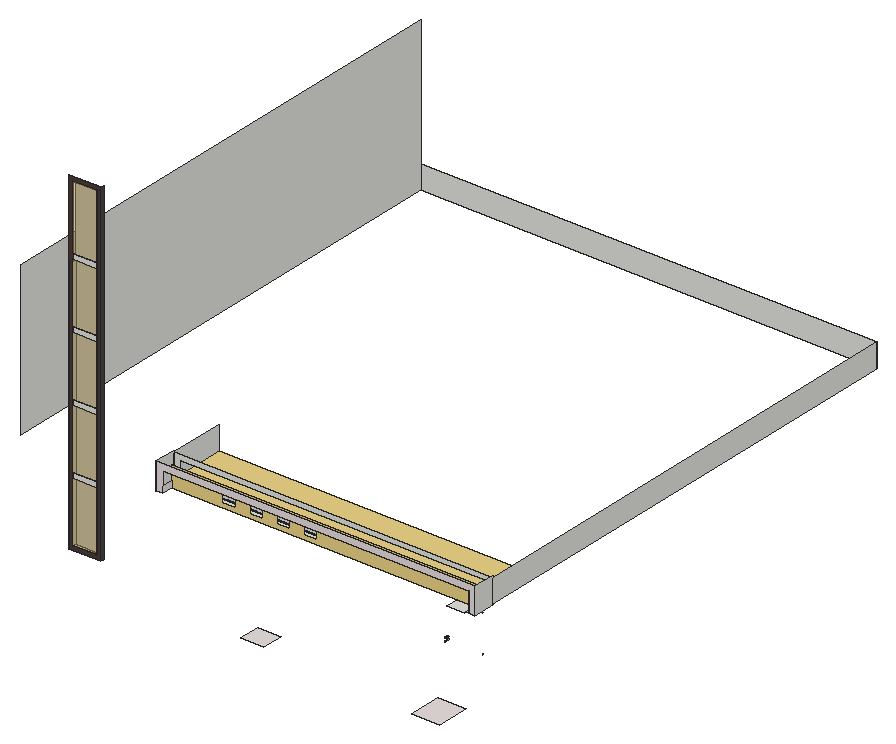
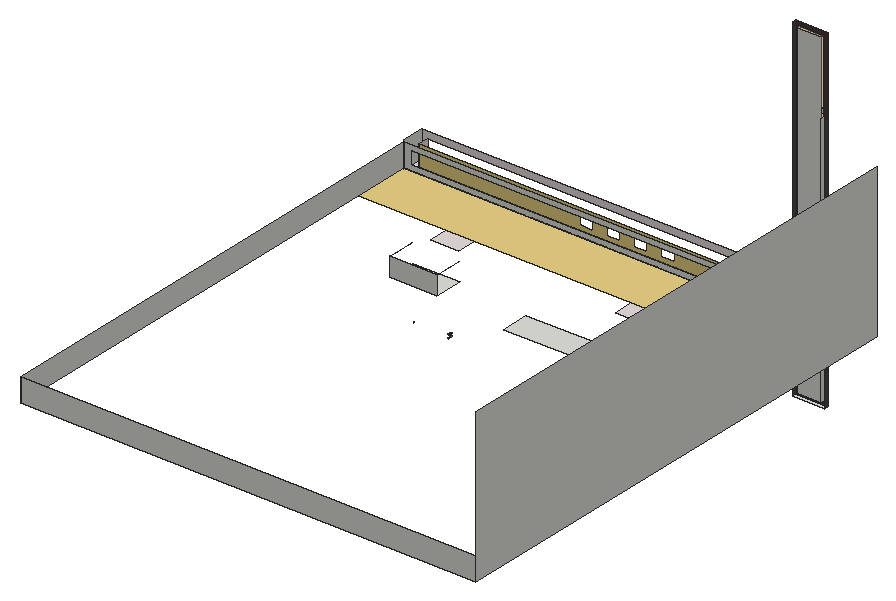
# SketchUp Ruby script. Lengths in inches.
U = 1.inch
M = Sketchup.active_model
def pt(a) = Geom::Point3d.new(a.map { |v| v * U })
def face(e, loops, mat)
  f = e.add_face(loops[0].map { |a| pt(a) })
  loops[1..].each { |l| e.add_face(l.map { |a| pt(a) }).erase! }
  f.material = f.back_material = mat if mat
  f
end
# faces: each face lists its corners as indices into pts; further lists are holes
def faces(e, pts, list, mat = nil) = list.each { |f| face(e, (f[0].is_a?(Array) ? f : [f]).map { |l| l.map { |i| pts[i] } }, mat) }
# xy, xz, yz: faces in a plane at the given z, y or x. An outline is a flat list of corners, or four numbers for a rectangle; further outlines are holes
def ring(l) = l.size == 4 ? [[l[0], l[1]], [l[2], l[1]], [l[2], l[3]], [l[0], l[3]]] : l.each_slice(2).to_a
def flat(e, list, mat, &to3) = list.each { |f| face(e, (f[0].is_a?(Array) ? f : [f]).map { |l| ring(l).map { |u, v| to3.(u, v) } }, mat) }
def xy(e, z, list, mat = nil) = flat(e, list, mat) { |x, y| [x, y, z] }
def xz(e, y, list, mat = nil) = flat(e, list, mat) { |x, z| [x, y, z] }
def yz(e, x, list, mat = nil) = flat(e, list, mat) { |y, z| [x, y, z] }
def lines(e, pts, list) = list.each { |a, b| e.add_line(pt(pts[a]), pt(pts[b])) }
# prism: a flat outline (further loops are holes) pulled along v
def prism(e, loops, v, mat = nil)
  f = face(e, loops, mat); d = Geom::Vector3d.new(v.map { |x| x * U })
  f.pushpull(f.normal.samedirection?(d) ? d.length : -d.length)
end
def box(e, o, s, mat = nil) = prism(e, [[o, [o[0] + s[0], o[1], o[2]], [o[0] + s[0], o[1] + s[1], o[2]], [o[0], o[1] + s[1], o[2]]]], [0, 0, s[2]], mat)
def at(x, y, z, deg = 0) = Geom::Transformation.translation(pt([x, y, z])) * Geom::Transformation.rotation(ORIGIN, Z_AXIS, deg.degrees)
def axes(o, x, y, z) = Geom::Transformation.new([*x, 0, *y, 0, *z, 0, *pt(o).to_a, 1])
def part(name) = M.definitions.add(name)
# library, detail: a bought-in or finely detailed component or shape, given as its bounding box
def library(name, o, s) = part(name).tap { |d| box(d.entities, o, s) }
def detail(e, o, s) = box(e.add_group.entities, o, s)
def put(e, d, t, mat = nil) = e.add_instance(d, t).tap { |i| i.material = mat if mat }
def group(e, t, mat = nil) = e.add_group.tap { |g| g.transformation = t; g.material = mat if mat }.entities
root = M.entities
M.materials.add("Generic\#1").color = [73, 71, 71]
M.materials.add("Generic\#2").color = [78, 57, 57]
M.materials.add("Generic\#3").color = [235, 210, 133]
M.materials.add("Generic\#5").color = [232, 222, 222]
M.materials.add("Material \#1").color = [140, 140, 140]
M.materials.add("[Translucent Glass Gray]").color = [186, 161, 89]
M.materials["[Translucent Glass Gray]"].alpha = 0.5
c1 = library("3DGeom~14_Defintion",[-102.17,352.37,-727.27],[204.35,204.35,1000])
c2 = library("3DGeom~1_Defintion",[-60.87,347.29,-704.08],[121.74,121.75,1000])
xy(root,34.35,[[371.22,117.13,371.16,117.15,371.23,117.15],[371.22,117.13,371.23,117.15,371.29,117.15],[371.22,117.13,371.29,117.15,371.29,117.13],[371.29,117.13,371.29,117.15,371.35,117.17],[371.29,117.13,371.35,117.17,371.36,117.15],
  [371.16,117.15,371.1,117.19,371.17,117.17],[371.16,117.15,371.17,117.17,371.23,117.15],[371.36,117.15,371.35,117.17,371.4,117.2],[371.36,117.15,371.4,117.2,371.42,117.19],[371.17,117.17,371.1,117.19,371.12,117.2],
  [371.1,117.19,371.07,117.25,371.12,117.2],[371.42,117.19,371.4,117.2,371.43,117.25],[371.42,117.19,371.43,117.25,371.45,117.25],[371.12,117.2,371.07,117.25,371.08,117.25],[371.07,117.25,371.05,117.3125,371.08,117.25],
  [371.08,117.25,371.05,117.3125,371.07,117.3125],[371.43,117.25,371.44,117.3125,371.45,117.25],[371.45,117.25,371.44,117.3125,371.47,117.3125],[371.05,117.3125,371.07,117.375,371.07,117.3125],[371.07,117.3125,371.07,117.375,371.08,117.37],
  [371.44,117.3125,371.43,117.37,371.47,117.3125],[371.47,117.3125,371.43,117.37,371.45,117.375],[371.08,117.37,371.07,117.375,371.1,117.43],[371.08,117.37,371.1,117.43,371.12,117.42],[371.43,117.37,371.4,117.42,371.45,117.375],
  [371.45,117.375,371.4,117.42,371.42,117.43],[371.12,117.42,371.1,117.43,371.16,117.47],[371.12,117.42,371.16,117.47,371.17,117.46],[371.4,117.42,371.35,117.46,371.42,117.43],[371.42,117.43,371.35,117.46,371.36,117.47],
  [371.17,117.46,371.16,117.47,371.22,117.5],[371.17,117.46,371.22,117.5,371.23,117.48],[371.35,117.46,371.29,117.48,371.36,117.47],[371.36,117.47,371.29,117.48,371.29,117.5],[371.23,117.48,371.22,117.5,371.29,117.5],
  [371.23,117.48,371.29,117.5,371.29,117.48]],"Material \#1")
xy(root,34.36,[[371.22,117.13,371.17,117.17,371.16,117.15],[371.22,117.13,371.23,117.15,371.17,117.17],[371.22,117.13,371.29,117.13,371.23,117.15],[371.29,117.13,371.29,117.15,371.23,117.15],[371.29,117.13,371.36,117.15,371.29,117.15],
  [371.16,117.15,371.12,117.2,371.1,117.19],[371.16,117.15,371.17,117.17,371.12,117.2],[371.29,117.15,371.36,117.15,371.35,117.17],[371.36,117.15,371.42,117.19,371.35,117.17],[371.35,117.17,371.42,117.19,371.4,117.2],
  [371.1,117.19,371.08,117.25,371.07,117.25],[371.1,117.19,371.12,117.2,371.08,117.25],[371.42,117.19,371.45,117.25,371.4,117.2],[371.4,117.2,371.45,117.25,371.43,117.25],[371.07,117.25,371.07,117.3125,371.05,117.3125],
  [371.07,117.25,371.08,117.25,371.07,117.3125],[371.43,117.25,371.45,117.25,371.47,117.3125],[371.43,117.25,371.47,117.3125,371.44,117.3125],[371.05,117.3125,371.07,117.3125,371.08,117.37],[371.05,117.3125,371.08,117.37,371.07,117.375],
  [371.44,117.3125,371.45,117.375,371.43,117.37],[371.44,117.3125,371.47,117.3125,371.45,117.375],[371.08,117.37,371.12,117.42,371.07,117.375],[371.43,117.37,371.42,117.43,371.4,117.42],[371.43,117.37,371.45,117.375,371.42,117.43],
  [371.07,117.375,371.12,117.42,371.1,117.43],[371.12,117.42,371.17,117.46,371.1,117.43],[371.4,117.42,371.36,117.47,371.35,117.46],[371.4,117.42,371.42,117.43,371.36,117.47],[371.1,117.43,371.17,117.46,371.16,117.47],
  [371.17,117.46,371.23,117.48,371.16,117.47],[371.35,117.46,371.29,117.5,371.29,117.48],[371.35,117.46,371.36,117.47,371.29,117.5],[371.16,117.47,371.23,117.48,371.22,117.5],[371.23,117.48,371.29,117.48,371.22,117.5],
  [371.29,117.48,371.29,117.5,371.22,117.5]],"Material \#1")
xy(root,43.23,[[47.67,39.25,77.59,42.5]])
xy(root,45.88,[[399.32,0,424.88,30.0625],[231.59,10.375,252.46,30.0625]],"Generic\#5")
xy(root,46.93,[[51.37,39.25,73.89,42.5]])
xy(root,69.12,[[371.22,117.13,371.16,117.15,371.17,117.17],[371.22,117.13,371.17,117.17,371.23,117.15],[371.22,117.13,371.23,117.15,371.29,117.13],[371.29,117.13,371.23,117.15,371.29,117.15],[371.29,117.13,371.29,117.15,371.36,117.15],
  [371.16,117.15,371.1,117.19,371.12,117.2],[371.16,117.15,371.12,117.2,371.17,117.17],[371.29,117.15,371.35,117.17,371.36,117.15],[371.36,117.15,371.35,117.17,371.42,117.19],[371.35,117.17,371.4,117.2,371.42,117.19],
  [371.1,117.19,371.07,117.25,371.08,117.25],[371.1,117.19,371.08,117.25,371.12,117.2],[371.42,117.19,371.4,117.2,371.45,117.25],[371.4,117.2,371.43,117.25,371.45,117.25],[371.07,117.25,371.05,117.3125,371.07,117.3125],
  [371.07,117.25,371.07,117.3125,371.08,117.25],[371.43,117.25,371.44,117.3125,371.47,117.3125],[371.43,117.25,371.47,117.3125,371.45,117.25],[371.05,117.3125,371.07,117.375,371.08,117.37],[371.05,117.3125,371.08,117.37,371.07,117.3125],
  [371.44,117.3125,371.43,117.37,371.45,117.375],[371.44,117.3125,371.45,117.375,371.47,117.3125],[371.08,117.37,371.07,117.375,371.12,117.42],[371.43,117.37,371.4,117.42,371.42,117.43],[371.43,117.37,371.42,117.43,371.45,117.375],
  [371.07,117.375,371.1,117.43,371.12,117.42],[371.12,117.42,371.1,117.43,371.17,117.46],[371.4,117.42,371.35,117.46,371.36,117.47],[371.4,117.42,371.36,117.47,371.42,117.43],[371.1,117.43,371.16,117.47,371.17,117.46],
  [371.17,117.46,371.16,117.47,371.23,117.48],[371.35,117.46,371.29,117.48,371.29,117.5],[371.35,117.46,371.29,117.5,371.36,117.47],[371.16,117.47,371.22,117.5,371.23,117.48],[371.23,117.48,371.22,117.5,371.29,117.48],
  [371.29,117.48,371.22,117.5,371.29,117.5]],"Material \#1")
xy(root,69.13,[[371.22,117.13,371.23,117.15,371.16,117.15],[371.22,117.13,371.29,117.13,371.29,117.15],[371.22,117.13,371.29,117.15,371.23,117.15],[371.29,117.13,371.35,117.17,371.29,117.15],[371.29,117.13,371.36,117.15,371.35,117.17],
  [371.16,117.15,371.17,117.17,371.1,117.19],[371.16,117.15,371.23,117.15,371.17,117.17],[371.36,117.15,371.4,117.2,371.35,117.17],[371.36,117.15,371.42,117.19,371.4,117.2],[371.17,117.17,371.12,117.2,371.1,117.19],
  [371.1,117.19,371.12,117.2,371.07,117.25],[371.42,117.19,371.43,117.25,371.4,117.2],[371.42,117.19,371.45,117.25,371.43,117.25],[371.12,117.2,371.08,117.25,371.07,117.25],[371.07,117.25,371.08,117.25,371.05,117.3125],
  [371.08,117.25,371.07,117.3125,371.05,117.3125],[371.43,117.25,371.45,117.25,371.44,117.3125],[371.45,117.25,371.47,117.3125,371.44,117.3125],[371.05,117.3125,371.07,117.3125,371.07,117.375],[371.07,117.3125,371.08,117.37,371.07,117.375],
  [371.44,117.3125,371.47,117.3125,371.43,117.37],[371.47,117.3125,371.45,117.375,371.43,117.37],[371.08,117.37,371.1,117.43,371.07,117.375],[371.08,117.37,371.12,117.42,371.1,117.43],[371.43,117.37,371.45,117.375,371.4,117.42],
  [371.45,117.375,371.42,117.43,371.4,117.42],[371.12,117.42,371.16,117.47,371.1,117.43],[371.12,117.42,371.17,117.46,371.16,117.47],[371.4,117.42,371.42,117.43,371.35,117.46],[371.42,117.43,371.36,117.47,371.35,117.46],
  [371.17,117.46,371.22,117.5,371.16,117.47],[371.17,117.46,371.23,117.48,371.22,117.5],[371.35,117.46,371.36,117.47,371.29,117.48],[371.36,117.47,371.29,117.5,371.29,117.48],[371.23,117.48,371.29,117.5,371.22,117.5],
  [371.23,117.48,371.29,117.48,371.29,117.5]],"Material \#1")
xy(root,72.98,[[371.22,117.13,371.16,117.15,371.23,117.15],[371.22,117.13,371.23,117.15,371.29,117.15],[371.22,117.13,371.29,117.15,371.29,117.13],[371.29,117.13,371.29,117.15,371.35,117.17],[371.29,117.13,371.35,117.17,371.36,117.15],
  [371.16,117.15,371.1,117.19,371.17,117.17],[371.16,117.15,371.17,117.17,371.23,117.15],[371.36,117.15,371.35,117.17,371.4,117.2],[371.36,117.15,371.4,117.2,371.42,117.19],[371.17,117.17,371.1,117.19,371.12,117.2],
  [371.1,117.19,371.07,117.25,371.12,117.2],[371.42,117.19,371.4,117.2,371.43,117.25],[371.42,117.19,371.43,117.25,371.45,117.25],[371.12,117.2,371.07,117.25,371.08,117.25],[371.07,117.25,371.05,117.3125,371.08,117.25],
  [371.08,117.25,371.05,117.3125,371.07,117.3125],[371.43,117.25,371.44,117.3125,371.45,117.25],[371.45,117.25,371.44,117.3125,371.47,117.3125],[371.05,117.3125,371.07,117.375,371.07,117.3125],[371.07,117.3125,371.07,117.375,371.08,117.37],
  [371.44,117.3125,371.43,117.37,371.47,117.3125],[371.47,117.3125,371.43,117.37,371.45,117.375],[371.08,117.37,371.07,117.375,371.1,117.43],[371.08,117.37,371.1,117.43,371.12,117.42],[371.43,117.37,371.4,117.42,371.45,117.375],
  [371.45,117.375,371.4,117.42,371.42,117.43],[371.12,117.42,371.1,117.43,371.16,117.47],[371.12,117.42,371.16,117.47,371.17,117.46],[371.4,117.42,371.35,117.46,371.42,117.43],[371.42,117.43,371.35,117.46,371.36,117.47],
  [371.17,117.46,371.16,117.47,371.22,117.5],[371.17,117.46,371.22,117.5,371.23,117.48],[371.35,117.46,371.29,117.48,371.36,117.47],[371.36,117.47,371.29,117.48,371.29,117.5],[371.23,117.48,371.22,117.5,371.29,117.5],
  [371.23,117.48,371.29,117.5,371.29,117.48]],"Material \#1")
xy(root,73,[[371.22,117.13,371.17,117.17,371.16,117.15],[371.22,117.13,371.23,117.15,371.17,117.17],[371.22,117.13,371.29,117.13,371.23,117.15],[371.29,117.13,371.29,117.15,371.23,117.15],[371.29,117.13,371.36,117.15,371.29,117.15],
  [371.16,117.15,371.12,117.2,371.1,117.19],[371.16,117.15,371.17,117.17,371.12,117.2],[371.29,117.15,371.36,117.15,371.35,117.17],[371.36,117.15,371.42,117.19,371.35,117.17],[371.35,117.17,371.42,117.19,371.4,117.2],
  [371.1,117.19,371.08,117.25,371.07,117.25],[371.1,117.19,371.12,117.2,371.08,117.25],[371.42,117.19,371.45,117.25,371.4,117.2],[371.4,117.2,371.45,117.25,371.43,117.25],[371.07,117.25,371.07,117.3125,371.05,117.3125],
  [371.07,117.25,371.08,117.25,371.07,117.3125],[371.43,117.25,371.45,117.25,371.47,117.3125],[371.43,117.25,371.47,117.3125,371.44,117.3125],[371.05,117.3125,371.07,117.3125,371.08,117.37],[371.05,117.3125,371.08,117.37,371.07,117.375],
  [371.44,117.3125,371.45,117.375,371.43,117.37],[371.44,117.3125,371.47,117.3125,371.45,117.375],[371.08,117.37,371.12,117.42,371.07,117.375],[371.43,117.37,371.42,117.43,371.4,117.42],[371.43,117.37,371.45,117.375,371.42,117.43],
  [371.07,117.375,371.12,117.42,371.1,117.43],[371.12,117.42,371.17,117.46,371.1,117.43],[371.4,117.42,371.36,117.47,371.35,117.46],[371.4,117.42,371.42,117.43,371.36,117.47],[371.1,117.43,371.17,117.46,371.16,117.47],
  [371.17,117.46,371.23,117.48,371.16,117.47],[371.35,117.46,371.29,117.5,371.29,117.48],[371.35,117.46,371.36,117.47,371.29,117.5],[371.16,117.47,371.23,117.48,371.22,117.5],[371.23,117.48,371.29,117.48,371.22,117.5],
  [371.29,117.48,371.29,117.5,371.22,117.5]],"Material \#1")
xy(root,75.1,[[205.2,114.8125,268.45,141.3125]])
xy(root,81.34,[[330.35,114.8125,374.48,141.3125]])
xy(root,118.6875,[[399.88,39.9375,416.23,51.9375],[127.58,41.4375,127.58,61.6875,424.88,61.6875,424.88,41.4375,418.88,41.4375,418.88,51.9375,416.23,51.9375,416.23,55.875,399.88,55.875,399.88,51.9375,133.33,51.9375,133.33,41.4375],[416.23,41.4375,418.88,51.9375],[399.88,51.9375,411.67,55.875],[411.67,51.9375,416.23,55.875]])
xy(root,120,[[127.58,61.6875,424.88,114.8125]],"Generic\#3")
xz(root,39.25,[[[47.67,43.23,77.59,43.23,77.58,355.68,47.61,355.68,47.61,283.88],[51.37,46.93,51.32,283.88,51.3125,351.98,73.88,351.98,73.89,46.93]]],"Generic\#2")
xz(root,41.4375,[[127.58,118.6875,133.33,118.6875,133.33,137.61,418.88,137.61,418.88,118.6875,424.88,118.6875,424.88,143.5,127.58,143.5]],"Generic\#5")
xz(root,42.5,[[51.37,46.93,73.89,46.93,73.88,351.98,51.3125,351.98,51.32,283.88]])
xz(root,51.9375,[[[133.33,118.6875,418.88,137.61],[180.71,122.76,193.02,131.39],[205.96,122.76,218.27,131.39],[231.21,122.76,243.52,131.39],[256.46,122.76,268.77,131.39]]],"Generic\#3")
xz(root,61.6875,[[127.58,118.6875,424.88,120],[[127.58,120,424.88,141.9375],[133.33,124.55,418.88,137.61]]])
xz(root,116.5625,[[336.5,36.6875,336.51,36.83,336.51,36.6875],[336.51,36.6875,336.51,36.83,336.52,36.82],[337.93,36.6875,337.92,36.82,337.94,36.6875],[337.94,36.6875,337.92,36.82,337.93,36.83],[337.22,36.74,337.18,36.75,337.22,36.76],
  [337.22,36.74,337.22,36.76,337.26,36.76],[337.22,36.74,337.26,36.76,337.26,36.75],[337.18,36.75,337.14,36.76,337.18,36.76],[337.18,36.75,337.18,36.76,337.22,36.76],[337.26,36.75,337.26,36.76,337.3,36.77],
  [337.26,36.75,337.3,36.77,337.3,36.76],[337.14,36.76,337.1,36.78,337.14,36.77],[337.14,36.76,337.14,36.77,337.18,36.76],[337.3,36.76,337.3,36.77,337.33,36.79],[337.3,36.76,337.33,36.79,337.34,36.78],
  [337.14,36.77,337.1,36.78,337.1,36.79],[337.1,36.78,337.0625,36.8,337.1,36.79],[337.34,36.78,337.33,36.79,337.37,36.8125],[337.34,36.78,337.37,36.8125,337.375,36.8],[337.1,36.79,337.0625,36.8,337.07,36.8125],
  [337.0625,36.8,337.04,36.83,337.07,36.8125],[337.375,36.8,337.37,36.8125,337.39,36.84],[337.375,36.8,337.39,36.84,337.4,36.83],[337.07,36.8125,337.04,36.83,337.04,36.84],[336.52,36.82,336.51,36.83,336.54,36.95],
  [336.52,36.82,336.54,36.95,336.55,36.95],[337.92,36.82,337.88,36.95,337.93,36.83],[337.04,36.83,337.01,36.87,337.04,36.84],[337.4,36.83,337.39,36.84,337.41,36.87],[337.4,36.83,337.41,36.87,337.43,36.87],
  [337.93,36.83,337.88,36.95,337.9,36.95],[337.04,36.84,337.01,36.87,337.02,36.87],[337.01,36.87,336.99,36.91,337.02,36.87],[337.02,36.87,336.99,36.91,337.01,36.91],[337.41,36.87,337.43,36.91,337.43,36.87],
  [337.43,36.87,337.43,36.91,337.44,36.91],[336.99,36.91,336.98,36.95,337.01,36.91],[337.01,36.91,336.98,36.95,336.99,36.95],[337.43,36.91,337.44,36.95,337.44,36.91],[337.44,36.91,337.44,36.95,337.45,36.95],
  [336.54,36.95,336.6,37.07,336.55,36.95],[336.55,36.95,336.6,37.07,336.61,37.0625],[336.98,36.95,336.98,37,336.99,36.95],[336.99,36.95,336.98,37,336.99,37],[337.44,36.95,337.45,36.99,337.45,36.95],
  [337.45,36.95,337.45,36.99,337.46,36.99],[337.88,36.95,337.83,37.0625,337.9,36.95],[337.9,36.95,337.83,37.0625,337.84,37.07],[337.45,36.99,337.44,37.03,337.46,36.99],[337.46,36.99,337.44,37.03,337.45,37.04],
  [336.98,37,336.98,37.04,336.99,37],[336.99,37,336.98,37.04,336.99,37.03],[336.99,37.03,336.98,37.04,336.99,37.08],[336.99,37.03,336.99,37.08,337.01,37.07],[337.44,37.03,337.43,37.07,337.45,37.04],
  [337.45,37.04,337.43,37.07,337.44,37.08],[336.61,37.0625,336.6,37.07,336.67,37.18],[336.61,37.0625,336.67,37.18,336.68,37.17],[337.83,37.0625,337.76,37.17,337.84,37.07],[337.01,37.07,336.99,37.08,337.01,37.12],
  [337.01,37.07,337.01,37.12,337.02,37.11],[337.43,37.07,337.41,37.11,337.44,37.08],[337.84,37.07,337.76,37.17,337.77,37.18],[337.44,37.08,337.41,37.11,337.43,37.12],[337.02,37.11,337.01,37.12,337.04,37.15],
  [337.02,37.11,337.04,37.15,337.04,37.14],[337.41,37.11,337.39,37.14,337.43,37.12],[337.43,37.12,337.39,37.14,337.4,37.15],[337.04,37.14,337.04,37.15,337.0625,37.18],[337.04,37.14,337.0625,37.18,337.07,37.17],
  [337.39,37.14,337.37,37.17,337.4,37.15],[337.4,37.15,337.37,37.17,337.375,37.18],[336.68,37.17,336.67,37.18,336.75,37.27],[336.68,37.17,336.75,37.27,336.76,37.26],[337.07,37.17,337.0625,37.18,337.1,37.21],
  [337.07,37.17,337.1,37.21,337.1,37.2],[337.37,37.17,337.33,37.2,337.375,37.18],[337.76,37.17,337.68,37.26,337.77,37.18],[337.375,37.18,337.33,37.2,337.34,37.21],[337.77,37.18,337.68,37.26,337.68,37.27],
  [337.1,37.2,337.1,37.21,337.14,37.23],[337.1,37.2,337.14,37.23,337.14,37.21],[337.33,37.2,337.3,37.21,337.34,37.21],[337.14,37.21,337.14,37.23,337.18,37.24],[337.14,37.21,337.18,37.24,337.18,37.23],
  [337.3,37.21,337.26,37.23,337.3,37.23],[337.3,37.21,337.3,37.23,337.34,37.21],[337.18,37.23,337.18,37.24,337.22,37.24],[337.18,37.23,337.22,37.24,337.22,37.23],[337.22,37.23,337.22,37.24,337.26,37.24],
  [337.22,37.23,337.26,37.24,337.26,37.23],[337.26,37.23,337.26,37.24,337.3,37.23],[336.76,37.26,336.75,37.27,336.85,37.34],[336.76,37.26,336.85,37.34,336.86,37.33],[337.68,37.26,337.58,37.33,337.68,37.27],
  [337.68,37.27,337.58,37.33,337.58,37.34],[336.86,37.33,336.85,37.34,336.97,37.4],[336.86,37.33,336.97,37.4,336.97,37.38],[337.58,37.33,337.47,37.38,337.58,37.34],[337.58,37.34,337.47,37.38,337.47,37.4],
  [336.97,37.38,336.97,37.4,337.09,37.43],[336.97,37.38,337.09,37.43,337.09,37.42],[337.47,37.38,337.35,37.42,337.47,37.4],[337.47,37.4,337.35,37.42,337.35,37.43],[337.09,37.42,337.09,37.43,337.22,37.44],
  [337.09,37.42,337.22,37.44,337.22,37.43],[337.35,37.42,337.22,37.43,337.35,37.43],[337.22,37.43,337.22,37.44,337.35,37.43]],"Material \#1")
xz(root,118.74,[[336.5,36.6875,336.51,36.6875,336.51,36.83],[336.51,36.6875,336.52,36.82,336.51,36.83],[337.93,36.6875,337.94,36.6875,337.92,36.82],[337.94,36.6875,337.93,36.83,337.92,36.82],[337.22,36.74,337.22,36.76,337.18,36.75],
  [337.22,36.74,337.26,36.75,337.26,36.76],[337.22,36.74,337.26,36.76,337.22,36.76],[337.18,36.75,337.18,36.76,337.14,36.76],[337.18,36.75,337.22,36.76,337.18,36.76],[337.26,36.75,337.3,36.76,337.3,36.77],
  [337.26,36.75,337.3,36.77,337.26,36.76],[337.14,36.76,337.14,36.77,337.1,36.78],[337.14,36.76,337.18,36.76,337.14,36.77],[337.3,36.76,337.33,36.79,337.3,36.77],[337.3,36.76,337.34,36.78,337.33,36.79],
  [337.14,36.77,337.1,36.79,337.1,36.78],[337.1,36.78,337.1,36.79,337.0625,36.8],[337.34,36.78,337.37,36.8125,337.33,36.79],[337.34,36.78,337.375,36.8,337.37,36.8125],[337.1,36.79,337.07,36.8125,337.0625,36.8],
  [337.0625,36.8,337.07,36.8125,337.04,36.83],[337.375,36.8,337.39,36.84,337.37,36.8125],[337.375,36.8,337.4,36.83,337.39,36.84],[337.07,36.8125,337.04,36.84,337.04,36.83],[336.52,36.82,336.54,36.95,336.51,36.83],
  [336.52,36.82,336.55,36.95,336.54,36.95],[337.92,36.82,337.93,36.83,337.88,36.95],[337.04,36.83,337.04,36.84,337.01,36.87],[337.4,36.83,337.41,36.87,337.39,36.84],[337.4,36.83,337.43,36.87,337.41,36.87],
  [337.93,36.83,337.9,36.95,337.88,36.95],[337.04,36.84,337.02,36.87,337.01,36.87],[337.01,36.87,337.02,36.87,336.99,36.91],[337.02,36.87,337.01,36.91,336.99,36.91],[337.41,36.87,337.43,36.87,337.43,36.91],
  [337.43,36.87,337.44,36.91,337.43,36.91],[336.99,36.91,337.01,36.91,336.98,36.95],[337.01,36.91,336.99,36.95,336.98,36.95],[337.43,36.91,337.44,36.91,337.44,36.95],[337.44,36.91,337.45,36.95,337.44,36.95],
  [336.54,36.95,336.55,36.95,336.6,37.07],[336.55,36.95,336.61,37.0625,336.6,37.07],[336.98,36.95,336.99,36.95,336.98,37],[336.99,36.95,336.99,37,336.98,37],[337.44,36.95,337.45,36.95,337.45,36.99],
  [337.45,36.95,337.46,36.99,337.45,36.99],[337.88,36.95,337.9,36.95,337.83,37.0625],[337.9,36.95,337.84,37.07,337.83,37.0625],[337.45,36.99,337.46,36.99,337.44,37.03],[337.46,36.99,337.45,37.04,337.44,37.03],
  [336.98,37,336.99,37,336.98,37.04],[336.99,37,336.99,37.03,336.98,37.04],[336.99,37.03,336.99,37.08,336.98,37.04],[336.99,37.03,337.01,37.07,336.99,37.08],[337.44,37.03,337.45,37.04,337.43,37.07],
  [337.45,37.04,337.44,37.08,337.43,37.07],[336.61,37.0625,336.67,37.18,336.6,37.07],[336.61,37.0625,336.68,37.17,336.67,37.18],[337.83,37.0625,337.84,37.07,337.76,37.17],[337.01,37.07,337.01,37.12,336.99,37.08],
  [337.01,37.07,337.02,37.11,337.01,37.12],[337.43,37.07,337.44,37.08,337.41,37.11],[337.84,37.07,337.77,37.18,337.76,37.17],[337.44,37.08,337.43,37.12,337.41,37.11],[337.02,37.11,337.04,37.15,337.01,37.12],
  [337.02,37.11,337.04,37.14,337.04,37.15],[337.41,37.11,337.43,37.12,337.39,37.14],[337.43,37.12,337.4,37.15,337.39,37.14],[337.04,37.14,337.0625,37.18,337.04,37.15],[337.04,37.14,337.07,37.17,337.0625,37.18],
  [337.39,37.14,337.4,37.15,337.37,37.17],[337.4,37.15,337.375,37.18,337.37,37.17],[336.68,37.17,336.75,37.27,336.67,37.18],[336.68,37.17,336.76,37.26,336.75,37.27],[337.07,37.17,337.1,37.21,337.0625,37.18],
  [337.07,37.17,337.1,37.2,337.1,37.21],[337.37,37.17,337.375,37.18,337.33,37.2],[337.76,37.17,337.77,37.18,337.68,37.26],[337.375,37.18,337.34,37.21,337.33,37.2],[337.77,37.18,337.68,37.27,337.68,37.26],
  [337.1,37.2,337.14,37.21,337.14,37.23],[337.1,37.2,337.14,37.23,337.1,37.21],[337.33,37.2,337.34,37.21,337.3,37.21],[337.14,37.21,337.18,37.23,337.18,37.24],[337.14,37.21,337.18,37.24,337.14,37.23],
  [337.3,37.21,337.3,37.23,337.26,37.23],[337.3,37.21,337.34,37.21,337.3,37.23],[337.18,37.23,337.22,37.23,337.22,37.24],[337.18,37.23,337.22,37.24,337.18,37.24],[337.22,37.23,337.26,37.23,337.26,37.24],
  [337.22,37.23,337.26,37.24,337.22,37.24],[337.26,37.23,337.3,37.23,337.26,37.24],[336.76,37.26,336.85,37.34,336.75,37.27],[336.76,37.26,336.86,37.33,336.85,37.34],[337.68,37.26,337.68,37.27,337.58,37.33],
  [337.68,37.27,337.58,37.34,337.58,37.33],[336.86,37.33,336.97,37.4,336.85,37.34],[336.86,37.33,336.97,37.38,336.97,37.4],[337.58,37.33,337.58,37.34,337.47,37.38],[337.58,37.34,337.47,37.4,337.47,37.38],
  [336.97,37.38,337.09,37.42,337.09,37.43],[336.97,37.38,337.09,37.43,336.97,37.4],[337.47,37.38,337.47,37.4,337.35,37.42],[337.47,37.4,337.35,37.43,337.35,37.42],[337.09,37.42,337.22,37.43,337.22,37.44],
  [337.09,37.42,337.22,37.44,337.09,37.43],[337.35,37.42,337.35,37.43,337.22,37.43],[337.22,37.43,337.35,37.43,337.22,37.44]],"Material \#1")
xz(root,141.3125,[[330.35,81.34,374.48,98.9]])
xz(root,508.6875,[[0,120,424.88,141.9375]])
yz(root,0,[[42.5,120,508.6875,261.9375]])
yz(root,127.58,[[41.4375,118.6875,61.6875,143.5],[61.6875,120,114.8125,141.9375]])
yz(root,133.33,[[41.4375,118.6875,51.9375,124.55]],"Generic\#5")
yz(root,418.88,[[41.4375,118.6875,51.9375,137.61]],"Generic\#5")
yz(root,424.88,[[41.4375,118.6875,61.6875,143.5],[61.6875,120,508.6875,141.9375]])
p = [[337.16,116.56,37.05],[337.16,116.59,37.05],[337.23,116.59,36.91],[337.23,116.56,36.91],[337.25,116.59,36.88],[337.25,116.5625,36.88],
  [337.26,116.6,36.86],[337.26,116.57,36.86],[337.28,116.56,36.9375],[337.28,116.59,36.9375],[337.2,116.59,37.08],[337.2,116.56,37.08],
  [337.29,116.6,36.87],[337.29,116.57,36.87],[337.3125,116.6,36.88],[337.3125,116.57,36.88],[337.3,116.59,36.91],[337.3,116.5625,36.91],
  [337.16,118.74,37.05],[337.23,118.74,36.91],[337.23,118.71,36.91],[337.16,118.71,37.05],[337.25,118.74,36.88],[337.25,118.71,36.88],
  [337.26,118.73,36.86],[337.26,118.7,36.86],[337.28,118.74,36.9375],[337.2,118.74,37.08],[337.2,118.71,37.08],[337.28,118.71,36.9375],
  [337.29,118.73,36.87],[337.29,118.7,36.87],[337.3125,118.73,36.88],[337.3125,118.7,36.88],[337.3,118.74,36.91],[337.3,118.71,36.91],
  [337.14,116.5625,37.07],[337.14,116.59,37.07],[337.14,118.74,37.07],[337.14,118.71,37.07],[337.18,116.57,37.13],[337.18,116.6,37.13],
  [337.15,116.6,37.12],[337.15,116.57,37.12],[337.125,116.6,37.1],[337.125,116.57,37.1],[337.19,116.59,37.1],[337.19,116.5625,37.1],
  [337.18,118.73,37.13],[337.15,118.73,37.12],[337.15,118.7,37.12],[337.18,118.7,37.13],[337.125,118.73,37.1],[337.125,118.7,37.1],
  [337.19,118.74,37.1],[337.19,118.71,37.1],[47.61,42.5,283.88],[47.67,42.5,43.23],[47.67,39.25,43.23],[47.61,39.25,283.88],
  [77.59,42.5,43.23],[77.58,42.5,355.68],[77.58,39.25,355.68],[77.59,39.25,43.23],[51.37,42.5,46.93],[51.32,42.5,283.88],
  [51.32,39.25,283.88],[51.37,39.25,46.93],[73.88,42.5,351.98],[73.89,42.5,46.93],[73.89,39.25,46.93],[73.88,39.25,351.98],
  [330.35,114.8125,98.9],[330.35,141.3125,98.9],[374.48,114.8125,98.9],[374.48,141.3125,98.9],[133.33,41.4375,118.6875],[133.33,41.4375,118.55]]
faces(root,p,[[0,1,2],[2,3,0],[3,2,4],[4,5,3],[5,4,6],[6,7,5],[8,9,10],[10,11,8],
  [7,6,12],[12,13,7],[13,12,14],[14,15,13],[15,14,16],[16,17,15],[17,16,9],[9,8,17],
  [18,19,20],[20,21,18],[19,22,23],[23,20,19],[22,24,25],[25,23,22],[26,27,28],[28,29,26],
  [24,30,31],[31,25,24],[30,32,33],[33,31,30],[32,34,35],[35,33,32],[34,26,29],[29,35,34],
  [36,37,1],[1,0,36],[38,18,21],[21,39,38],[40,41,42],[42,43,40],[43,42,44],[44,45,43],
  [45,44,37],[37,36,45],[11,10,46],[46,47,11],[47,46,41],[41,40,47],[48,49,50],[50,51,48],
  [49,52,53],[53,50,49],[52,38,39],[39,53,52],[27,54,55],[55,28,27],[54,48,51],[51,55,54]],"Material \#1")
faces(root,p,[[56,57,58,59],[60,61,62,63]],"Generic\#1")
faces(root,p,[[64,65,66,67],[68,69,70,71]])
lines(root,p,[[72,73],[74,75],[76,77]])
put(root,c1,axes([337.22,118.4,32.4],[0.00363,0,0],[0,0,0.00378],[0,0.0033,0]),"Material \#1")
put(root,c2,axes([337.22,118.4,32.4],[0.00404,0,0],[0,0,0.00421],[0,0.00368,0]),"Material \#1")
g1 = group(root,at(51.3125,39.25,46.93))
xz(g1,0,[[0.043,56.447,22.579,61.01],[0.03,117.457,22.577,122.02],[0.016,178.467,22.575,183.029],[0.004,239.477,22.573,244.039]])
xz(g1,0,[[0.057,0,22.581,0,22.579,56.447,0.043,56.447],[0.043,61.01,22.579,61.01,22.577,117.457,0.03,117.457],[0.03,122.02,22.577,122.02,22.575,178.467,0.016,178.467],[0.016,183.029,22.575,183.029,22.573,239.477,0.004,239.477,0.004,236.949],[0.004,244.039,22.573,244.039,22.571,305.049,0,305.049]],"[Translucent Glass Gray]")
p = [[0.016,0,183.029],[0.004,0,183.029],[0.03,0,122.02],[0.006,0,122.02],[0.004,0,244.039],[0.002,0,244.039],
  [0.043,0,61.01],[0.008,0,61.01],[0.057,0,0],[0.01,0,0]]
lines(g1,p,[[0,1],[2,3],[4,5],[6,7],[8,9]])
